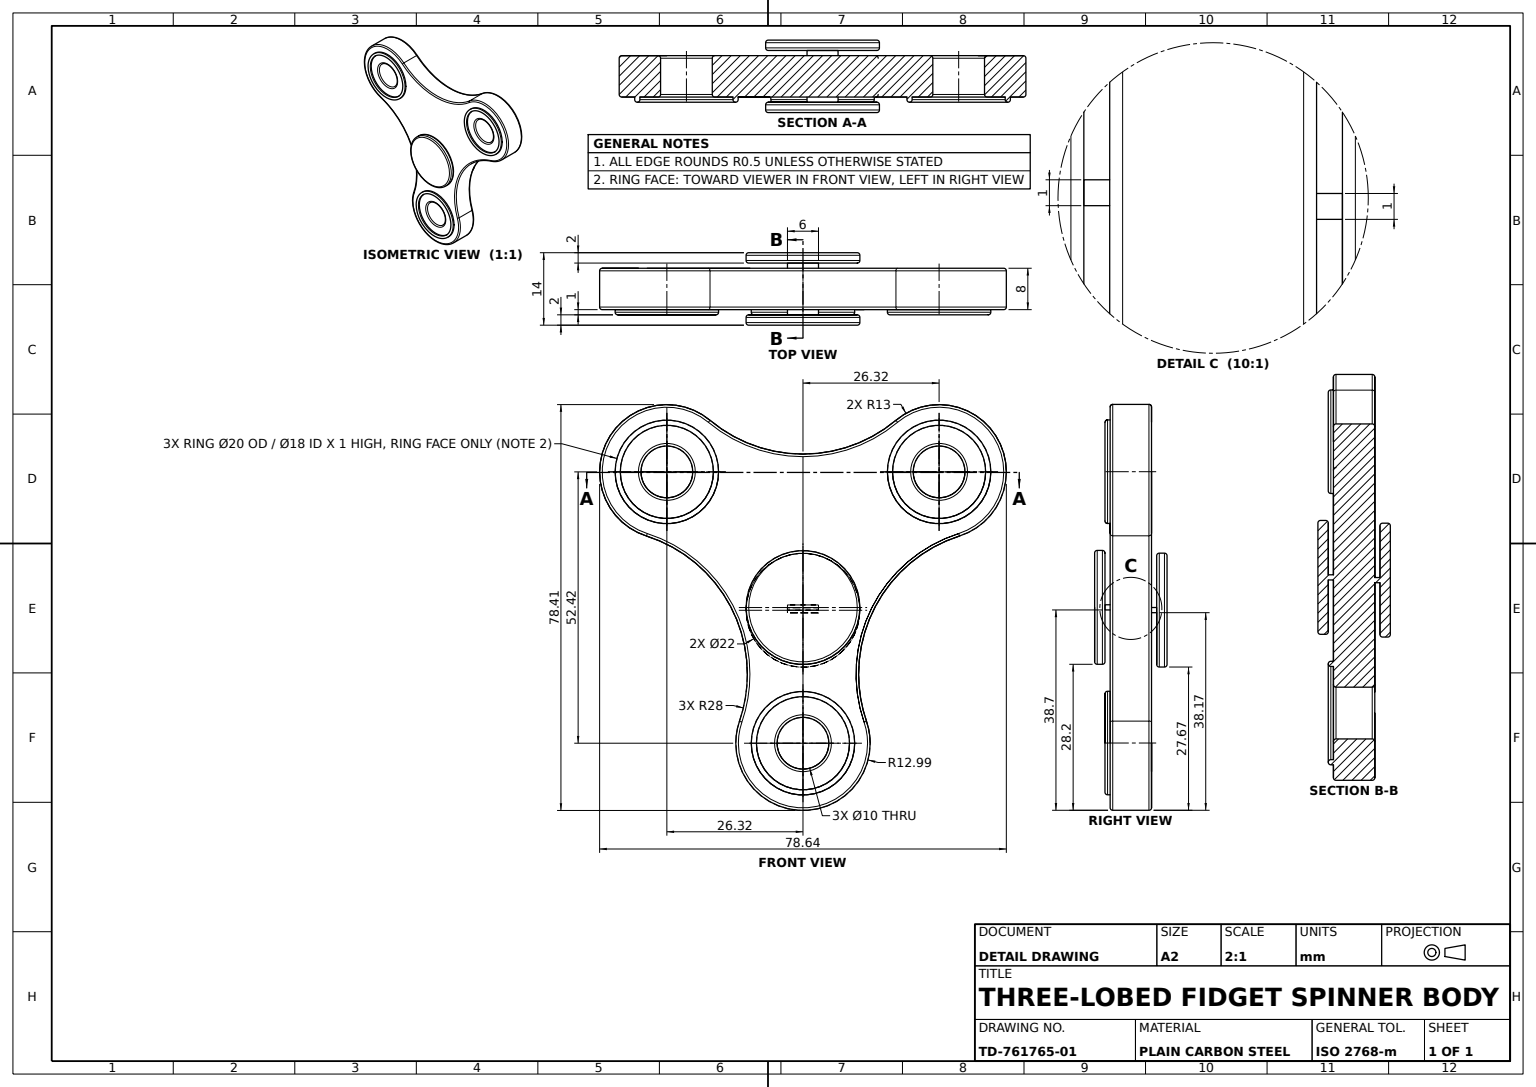
solid
v1 (-3,1.181214,0)
v2 (3,1.181214,0)
e1 v1 v2 LINE
v3 (3,1.181214,-1)
e2 v3 v2 LINE
v4 (-3,1.181214,-1)
e3 v4 v3 LINE
e4 v4 v1 LINE
face PLANE(AX(P(3,1.181214,-1),D(0,-1,0),D(0,0,-1))) rev [e1 -e2 -e3 e4]
v5 (35.319974,27.417425,8)
v6 (17.319974,27.417425,8)
e5 v5 v6 CIRCLE(AX(P(26.319974,27.417425,8),D(0,0,-1),D(1,0,0)),9)
e6 v6 v5 CIRCLE(AX(P(26.319974,27.417425,8),D(0,0,-1),D(1,0,0)),9)
v7 (20.819974,27.417425,8)
v8 (31.819974,27.417425,8)
e7 v7 v8 CIRCLE(AX(P(26.319974,27.417425,8),D(0,0,-1),D(1,0,0)),5.5)
e8 v8 v7 CIRCLE(AX(P(26.319974,27.417425,8),D(0,0,-1),D(1,0,0)),5.5)
face PLANE(AX(P(-32.539106,7.883547,8),D(0,0,1),D(1,0,0))) [-e5 -e6] [e7 e8]
v9 (16.819974,27.417425,9)
v10 (35.819974,27.417425,9)
e9 v9 v10 CIRCLE(AX(P(26.319974,27.417425,9),D(0,0,1),D(1,0,0)),9.5)
v11 (16.319974,27.417425,8.5)
e10 v11 v9 CIRCLE(AX(P(16.819974,27.417425,8.5),D(0,1,0),D(-1,0,0)),0.5)
v12 (36.319974,27.417425,8.5)
e11 v12 v11 CIRCLE(AX(P(26.319974,27.417425,8.5),D(0,0,-1),D(1,0,0)),10)
e12 v12 v10 CIRCLE(AX(P(35.819974,27.417425,8.5),D(0,-1,0),D(0,0,-1)),0.5)
face TORUS(AX(P(26.319974,27.417425,8.5),D(0,0,1),D(1,0,0)),9.5,0.5) [-e9 -e10 -e11 e12]
v13 (21.319974,27.417425,7.5)
e13 v7 v13 CIRCLE(AX(P(20.819974,27.417425,7.5),D(0,1,0),D(-1,0,0)),0.5)
v14 (31.319974,27.417425,7.5)
e14 v14 v13 CIRCLE(AX(P(26.319974,27.417425,7.5),D(0,0,1),D(1,0,0)),5)
e15 v8 v14 CIRCLE(AX(P(31.819974,27.417425,7.5),D(0,-1,0),D(0,0,-1)),0.5)
face TORUS(AX(P(26.319974,27.417425,7.5),D(0,0,1),D(1,0,0)),5.5,0.5) [-e7 e13 -e14 -e15]
v15 (11,0.681214,-1.5)
v16 (-11,0.681214,-1.5)
e16 v15 v16 CIRCLE(AX(P(0,0.681214,-1.5),D(0,0,-1),D(-1,0,0)),11)
v17 (10.5,0.681214,-1)
e17 v17 v15 CIRCLE(AX(P(10.5,0.681214,-1.5),D(0,1,0),D(-1,0,0)),0.5)
v18 (-10.5,0.681214,-1)
e18 v18 v17 CIRCLE(AX(P(0,0.681214,-1),D(0,0,1),D(-1,0,0)),10.5)
e19 v18 v16 CIRCLE(AX(P(-10.5,0.681214,-1.5),D(0,-1,0),D(0,0,-1)),0.5)
face TORUS(AX(P(0,0.681214,-1.5),D(0,0,-1),D(-1,0,0)),10.5,0.5) [-e16 -e17 -e18 e19]
v19 (-11,1.21,10.5)
v20 (-11,1.21,9.5)
e20 v19 v20 LINE
v21 (11,1.21,9.5)
e21 v20 v21 CIRCLE(AX(P(0,1.21,9.5),D(0,0,1),D(1,0,0)),11)
v22 (11,1.21,10.5)
e22 v22 v21 LINE
e23 v22 v19 CIRCLE(AX(P(0,1.21,10.5),D(0,0,-1),D(1,0,0)),11)
face CYL(AX(P(0,1.21,11),D(0,0,-1),D(-1,0,0)),11) [e20 e21 -e22 e23]
v23 (-10.258238,-11.650331,0)
v24 (-30.112128,15.506524,0)
e24 v23 v24 CIRCLE(AX(P(-38.758238,-11.650331,0),D(0,0,1),D(1,0,0)),28.5)
v25 (-10.758238,-11.650331,0.5)
e25 v25 v23 CIRCLE(AX(P(-10.258238,-11.650331,0.5),D(0,-1,0),D(0,0,-1)),0.5)
v26 (-30.263814,15.030088,0.5)
e26 v26 v25 CIRCLE(AX(P(-38.758238,-11.650331,0.5),D(0,0,-1),D(1,0,0)),28)
e27 v24 v26 CIRCLE(AX(P(-30.112128,15.506524,0.5),D(-0.952872102,0.303372309,0),D(-0.303372309,-0.952872102,0)),0.5)
face TORUS(AX(P(-38.758238,-11.650331,0.5),D(0,0,1),D(1,0,0)),28.5,0.5) [-e24 -e25 -e26 -e27]
v27 (-11,0.681214,-2.5)
e28 v27 v16 LINE
e29 v16 v15 CIRCLE(AX(P(0,0.681214,-1.5),D(0,0,-1),D(-1,0,0)),11)
v28 (11,0.681214,-2.5)
e30 v28 v15 LINE
e31 v28 v27 CIRCLE(AX(P(0,0.681214,-2.5),D(0,0,1),D(-1,0,0)),11)
face CYL(AX(P(0,0.681214,-3),D(0,0,1),D(1,0,0)),11) [e28 e29 -e30 e31]
v29 (-16.819974,27.417425,9)
v30 (-35.819974,27.417425,9)
e32 v29 v30 CIRCLE(AX(P(-26.319974,27.417425,9),D(0,0,1),D(1,0,0)),9.5)
v31 (-16.319974,27.417425,8.5)
e33 v31 v29 CIRCLE(AX(P(-16.819974,27.417425,8.5),D(0,-1,0),D(0,0,-1)),0.5)
v32 (-36.319974,27.417425,8.5)
e34 v32 v31 CIRCLE(AX(P(-26.319974,27.417425,8.5),D(0,0,-1),D(1,0,0)),10)
e35 v32 v30 CIRCLE(AX(P(-35.819974,27.417425,8.5),D(0,1,0),D(-1,0,0)),0.5)
face TORUS(AX(P(-26.319974,27.417425,8.5),D(0,0,1),D(1,0,0)),9.5,0.5) [-e32 -e33 -e34 e35]
v33 (11.811845,-20.931595,8)
v34 (30.112128,15.506524,8)
e36 v33 v34 CIRCLE(AX(P(38.758238,-11.650331,8),D(0,0,-1),D(1,0,0)),28.5)
v35 (12.284588,-20.768766,7.5)
e37 v35 v33 CIRCLE(AX(P(11.811845,-20.931595,7.5),D(0.325658377,-0.945487505,0),D(0.945487505,0.325658377,0)),0.5)
v36 (10.758238,-11.650331,7.5)
e38 v36 v35 CIRCLE(AX(P(38.758238,-11.650331,7.5),D(0,0,1),D(1,0,0)),28)
v37 (30.263814,15.030088,7.5)
e39 v37 v36 CIRCLE(AX(P(38.758238,-11.650331,7.5),D(0,0,1),D(1,0,0)),28)
e40 v34 v37 CIRCLE(AX(P(30.112128,15.506524,7.5),D(0.952872102,0.303372309,0),D(-0.303372309,0.952872102,0)),0.5)
face TORUS(AX(P(38.758238,-11.650331,7.5),D(0,0,1),D(1,0,0)),28.5,0.5) [-e36 -e37 -e38 -e39 -e40]
v38 (10.5,1.21,11)
e41 v22 v38 CIRCLE(AX(P(10.5,1.21,10.5),D(0,-1,0),D(0,0,-1)),0.5)
v39 (-10.5,1.21,11)
e42 v39 v38 CIRCLE(AX(P(0,1.21,11),D(0,0,1),D(1,0,0)),10.5)
e43 v19 v39 CIRCLE(AX(P(-10.5,1.21,10.5),D(0,1,0),D(-1,0,0)),0.5)
face TORUS(AX(P(0,1.21,10.5),D(0,0,1),D(1,0,0)),10.5,0.5) [-e23 e41 -e42 -e43]
v40 (-31.319974,27.417425,0.5)
v41 (-21.319974,27.417425,0.5)
e44 v40 v41 CIRCLE(AX(P(-26.319974,27.417425,0.5),D(0,0,-1),D(1,0,0)),5)
v42 (-21.319974,27.417425,7.5)
e45 v41 v42 LINE
v43 (-31.319974,27.417425,7.5)
e46 v42 v43 CIRCLE(AX(P(-26.319974,27.417425,7.5),D(0,0,1),D(1,0,0)),5)
e47 v40 v43 LINE
face CYL(AX(P(-26.319974,27.417425,0),D(0,0,1),D(1,0,0)),5) rev [e44 e45 e46 -e47]
v44 (-17.974616,37.385123,0.5)
v45 (-18.295592,37.00175,0)
e48 v44 v45 CIRCLE(AX(P(-18.295592,37.00175,0.5),D(-0.766746016,0.64195058,0),D(-0.64195058,-0.766746016,0)),0.5)
v46 (17.974616,37.385123,0.5)
e49 v46 v44 CIRCLE(AX(P(0,58.854012,0.5),D(0,0,-1),D(1,0,0)),28)
v47 (18.295592,37.00175,0)
e50 v46 v47 CIRCLE(AX(P(18.295592,37.00175,0.5),D(-0.766746016,-0.64195058,0),D(0.64195058,-0.766746016,0)),0.5)
e51 v45 v47 CIRCLE(AX(P(0,58.854012,0),D(0,0,1),D(1,0,0)),28.5)
face TORUS(AX(P(0,58.854012,0.5),D(0,0,1),D(1,0,0)),28.5,0.5) [-e48 -e49 e50 -e51]
v48 (3,0.181214,-1)
e52 v3 v48 LINE
v49 (-3,0.181214,-1)
e53 v48 v49 LINE
e54 v49 v4 LINE
e55 v17 v18 CIRCLE(AX(P(0,0.681214,-1),D(0,0,1),D(-1,0,0)),10.5)
face PLANE(AX(P(0,0.681214,-1),D(0,0,-1),D(-1,0,0))) rev [e52 e53 e54 e3] [e18 e55]
v50 (-30.263814,15.030088,7.5)
v51 (-30.112128,15.506524,8)
e56 v50 v51 CIRCLE(AX(P(-30.112128,15.506524,7.5),D(-0.952872102,0.303372309,0),D(-0.303372309,-0.952872102,0)),0.5)
v52 (-18.295592,37.00175,8)
e57 v52 v51 CIRCLE(AX(P(-26.319974,27.417425,8),D(0,0,1),D(1,0,0)),12.5)
v53 (-17.974616,37.385123,7.5)
e58 v52 v53 CIRCLE(AX(P(-18.295592,37.00175,7.5),D(-0.766746016,0.64195058,0),D(-0.64195058,-0.766746016,0)),0.5)
v54 (-39.319974,27.417425,7.5)
e59 v54 v53 CIRCLE(AX(P(-26.319974,27.417425,7.5),D(0,0,-1),D(1,0,0)),13)
e60 v50 v54 CIRCLE(AX(P(-26.319974,27.417425,7.5),D(0,0,-1),D(1,0,0)),13)
face TORUS(AX(P(-26.319974,27.417425,7.5),D(0,0,1),D(1,0,0)),12.5,0.5) [e56 -e57 e58 -e59 -e60]
v55 (16.319974,27.417425,8)
e61 v11 v55 LINE
v56 (36.319974,27.417425,8)
e62 v55 v56 CIRCLE(AX(P(26.319974,27.417425,8),D(0,0,1),D(1,0,0)),10)
e63 v12 v56 LINE
face CYL(AX(P(26.319974,27.417425,9),D(0,0,-1),D(-1,0,0)),10) [e61 e62 -e63 e11]
v57 (10,-25,8.5)
v58 (10,-25,8)
e64 v57 v58 LINE
v59 (-10,-25,8.5)
e65 v57 v59 CIRCLE(AX(P(0,-25,8.5),D(0,0,-1),D(1,0,0)),10)
v60 (-10,-25,8)
e66 v59 v60 LINE
e67 v60 v58 CIRCLE(AX(P(0,-25,8),D(0,0,1),D(1,0,0)),10)
face CYL(AX(P(0,-25,9),D(0,0,-1),D(-1,0,0)),10) [-e64 e65 e66 e67]
e68 v38 v39 CIRCLE(AX(P(0,1.21,11),D(0,0,1),D(1,0,0)),10.5)
e69 v19 v22 CIRCLE(AX(P(0,1.21,10.5),D(0,0,-1),D(1,0,0)),11)
face TORUS(AX(P(0,1.21,10.5),D(0,0,1),D(1,0,0)),10.5,0.5) [e43 -e68 -e41 -e69]
v61 (-11.811845,-20.931595,0)
v62 (-12.284588,-20.768766,0.5)
e70 v61 v62 CIRCLE(AX(P(-11.811845,-20.931595,0.5),D(0.325658377,0.945487505,0),D(-0.945487505,0.325658377,0)),0.5)
e71 v25 v62 CIRCLE(AX(P(-38.758238,-11.650331,0.5),D(0,0,-1),D(1,0,0)),28)
e72 v61 v23 CIRCLE(AX(P(-38.758238,-11.650331,0),D(0,0,1),D(1,0,0)),28.5)
face TORUS(AX(P(-38.758238,-11.650331,0.5),D(0,0,1),D(1,0,0)),28.5,0.5) [e70 -e71 e25 -e72]
e73 v50 v26 LINE
v63 (-12.284588,-20.768766,7.5)
e74 v63 v62 LINE
v64 (-10.758238,-11.650331,7.5)
e75 v63 v64 CIRCLE(AX(P(-38.758238,-11.650331,7.5),D(0,0,1),D(1,0,0)),28)
e76 v64 v50 CIRCLE(AX(P(-38.758238,-11.650331,7.5),D(0,0,1),D(1,0,0)),28)
face CYL(AX(P(-38.758238,-11.650331,8),D(0,0,-1),D(-1,0,0)),28) rev [e73 e26 e71 -e74 e75 e76]
v65 (12.992862,-25,7.5)
v66 (12.492862,-25,8)
e77 v65 v66 CIRCLE(AX(P(12.492862,-25,7.5),D(0,-1,0),D(0,0,-1)),0.5)
e78 v35 v65 CIRCLE(AX(P(0,-25,7.5),D(0,0,-1),D(1,0,0)),12.992862)
e79 v66 v33 CIRCLE(AX(P(0,-25,8),D(0,0,1),D(1,0,0)),12.492862)
face TORUS(AX(P(0,-25,7.5),D(0,0,1),D(1,0,0)),12.492862,0.5) [-e77 -e78 e37 -e79]
v67 (17.319974,27.417425,8.5)
e80 v67 v6 LINE
v68 (35.319974,27.417425,8.5)
e81 v68 v5 LINE
e82 v68 v67 CIRCLE(AX(P(26.319974,27.417425,8.5),D(0,0,1),D(1,0,0)),9)
face CYL(AX(P(26.319974,27.417425,9),D(0,0,-1),D(-1,0,0)),9) rev [e80 e6 -e81 e82]
v69 (-17.319974,27.417425,8.5)
v70 (-35.319974,27.417425,8.5)
e83 v69 v70 CIRCLE(AX(P(-26.319974,27.417425,8.5),D(0,0,1),D(1,0,0)),9)
v71 (-35.319974,27.417425,8)
e84 v70 v71 LINE
v72 (-17.319974,27.417425,8)
e85 v72 v71 CIRCLE(AX(P(-26.319974,27.417425,8),D(0,0,1),D(1,0,0)),9)
e86 v69 v72 LINE
face CYL(AX(P(-26.319974,27.417425,9),D(0,0,-1),D(-1,0,0)),9) rev [e83 e84 -e85 -e86]
v73 (31.319974,27.417425,0.5)
v74 (21.319974,27.417425,0.5)
e87 v73 v74 CIRCLE(AX(P(26.319974,27.417425,0.5),D(0,0,-1),D(1,0,0)),5)
e88 v74 v13 LINE
e89 v13 v14 CIRCLE(AX(P(26.319974,27.417425,7.5),D(0,0,1),D(1,0,0)),5)
e90 v73 v14 LINE
face CYL(AX(P(26.319974,27.417425,0),D(0,0,1),D(1,0,0)),5) rev [e87 e88 e89 -e90]
v75 (17.974616,37.385123,7.5)
e91 v53 v75 CIRCLE(AX(P(0,58.854012,7.5),D(0,0,1),D(1,0,0)),28)
v76 (18.295592,37.00175,8)
e92 v76 v52 CIRCLE(AX(P(0,58.854012,8),D(0,0,-1),D(1,0,0)),28.5)
e93 v76 v75 CIRCLE(AX(P(18.295592,37.00175,7.5),D(-0.766746016,-0.64195058,0),D(0.64195058,-0.766746016,0)),0.5)
face TORUS(AX(P(0,58.854012,7.5),D(0,0,1),D(1,0,0)),28.5,0.5) [-e91 -e58 -e92 e93]
e94 v43 v42 CIRCLE(AX(P(-26.319974,27.417425,7.5),D(0,0,1),D(1,0,0)),5)
e95 v41 v40 CIRCLE(AX(P(-26.319974,27.417425,0.5),D(0,0,-1),D(1,0,0)),5)
face CYL(AX(P(-26.319974,27.417425,0),D(0,0,1),D(1,0,0)),5) rev [e94 -e45 e95 e47]
v77 (-20.819974,27.417425,8)
v78 (-31.819974,27.417425,8)
e96 v77 v78 CIRCLE(AX(P(-26.319974,27.417425,8),D(0,0,-1),D(1,0,0)),5.5)
e97 v77 v42 CIRCLE(AX(P(-20.819974,27.417425,7.5),D(0,-1,0),D(0,0,-1)),0.5)
e98 v78 v43 CIRCLE(AX(P(-31.819974,27.417425,7.5),D(0,1,0),D(-1,0,0)),0.5)
face TORUS(AX(P(-26.319974,27.417425,7.5),D(0,0,1),D(1,0,0)),5.5,0.5) [-e96 e97 -e94 -e98]
v79 (-5.5,-25,8)
v80 (-5,-25,7.5)
e99 v79 v80 CIRCLE(AX(P(-5.5,-25,7.5),D(0,1,0),D(-1,0,0)),0.5)
v81 (5,-25,7.5)
e100 v81 v80 CIRCLE(AX(P(0,-25,7.5),D(0,0,1),D(1,0,0)),5)
v82 (5.5,-25,8)
e101 v82 v81 CIRCLE(AX(P(5.5,-25,7.5),D(0,-1,0),D(0,0,-1)),0.5)
e102 v79 v82 CIRCLE(AX(P(0,-25,8),D(0,0,-1),D(1,0,0)),5.5)
face TORUS(AX(P(0,-25,7.5),D(0,0,1),D(1,0,0)),5.5,0.5) [e99 -e100 -e101 -e102]
e103 v29 v69 CIRCLE(AX(P(-16.819974,27.417425,8.5),D(0,-1,0),D(0,0,-1)),0.5)
e104 v30 v70 CIRCLE(AX(P(-35.819974,27.417425,8.5),D(0,1,0),D(-1,0,0)),0.5)
face TORUS(AX(P(-26.319974,27.417425,8.5),D(0,0,1),D(1,0,0)),9.5,0.5) [-e83 -e103 e32 e104]
v83 (39.319974,27.417425,7.5)
v84 (38.819974,27.417425,8)
e105 v83 v84 CIRCLE(AX(P(38.819974,27.417425,7.5),D(0,-1,0),D(0,0,-1)),0.5)
e106 v75 v83 CIRCLE(AX(P(26.319974,27.417425,7.5),D(0,0,-1),D(1,0,0)),13)
e107 v84 v76 CIRCLE(AX(P(26.319974,27.417425,8),D(0,0,1),D(1,0,0)),12.5)
face TORUS(AX(P(26.319974,27.417425,7.5),D(0,0,1),D(1,0,0)),12.5,0.5) [-e105 -e106 -e93 -e107]
v85 (-16.319974,27.417425,8)
v86 (-36.319974,27.417425,8)
e108 v85 v86 CIRCLE(AX(P(-26.319974,27.417425,8),D(0,0,1),D(1,0,0)),10)
e109 v32 v86 LINE
e110 v31 v85 LINE
face CYL(AX(P(-26.319974,27.417425,9),D(0,0,-1),D(-1,0,0)),10) [e108 -e109 e34 e110]
v87 (-12.992862,-25,7.5)
e111 v87 v63 CIRCLE(AX(P(0,-25,7.5),D(0,0,-1),D(1,0,0)),12.992862)
v88 (-12.992862,-25,0.5)
e112 v62 v88 CIRCLE(AX(P(0,-25,0.5),D(0,0,1),D(1,0,0)),12.992862)
e113 v87 v88 LINE
face CYL(AX(P(0,-25,8),D(0,0,-1),D(-1,0,0)),12.992862) [e111 e74 e112 -e113]
e114 v10 v9 CIRCLE(AX(P(26.319974,27.417425,9),D(0,0,1),D(1,0,0)),9.5)
e115 v11 v12 CIRCLE(AX(P(26.319974,27.417425,8.5),D(0,0,-1),D(1,0,0)),10)
face TORUS(AX(P(26.319974,27.417425,8.5),D(0,0,1),D(1,0,0)),9.5,0.5) [e10 -e114 -e12 -e115]
v89 (-20.819974,27.417425,0)
e116 v41 v89 CIRCLE(AX(P(-20.819974,27.417425,0.5),D(0,-1,0),D(0,0,-1)),0.5)
v90 (-31.819974,27.417425,0)
e117 v40 v90 CIRCLE(AX(P(-31.819974,27.417425,0.5),D(0,1,0),D(-1,0,0)),0.5)
e118 v89 v90 CIRCLE(AX(P(-26.319974,27.417425,0),D(0,0,1),D(1,0,0)),5.5)
face TORUS(AX(P(-26.319974,27.417425,0.5),D(0,0,1),D(1,0,0)),5.5,0.5) [-e116 -e44 e117 -e118]
v91 (-39.319974,27.417425,0.5)
e119 v91 v26 CIRCLE(AX(P(-26.319974,27.417425,0.5),D(0,0,1),D(1,0,0)),13)
e120 v44 v91 CIRCLE(AX(P(-26.319974,27.417425,0.5),D(0,0,1),D(1,0,0)),13)
e121 v24 v45 CIRCLE(AX(P(-26.319974,27.417425,0),D(0,0,-1),D(1,0,0)),12.5)
face TORUS(AX(P(-26.319974,27.417425,0.5),D(0,0,1),D(1,0,0)),12.5,0.5) [-e119 -e120 e48 -e121 e27]
v92 (9,-25,8)
v93 (-9,-25,8)
e122 v92 v93 CIRCLE(AX(P(0,-25,8),D(0,0,-1),D(1,0,0)),9)
v94 (-9,-25,8.5)
e123 v94 v93 LINE
v95 (9,-25,8.5)
e124 v94 v95 CIRCLE(AX(P(0,-25,8.5),D(0,0,1),D(1,0,0)),9)
e125 v95 v92 LINE
face CYL(AX(P(0,-25,9),D(0,0,-1),D(-1,0,0)),9) rev [e122 -e123 e124 e125]
v96 (12.992862,-25,0.5)
e126 v65 v96 LINE
v97 (12.284588,-20.768766,0.5)
e127 v96 v97 CIRCLE(AX(P(0,-25,0.5),D(0,0,1),D(1,0,0)),12.992862)
e128 v35 v97 LINE
face CYL(AX(P(0,-25,8),D(0,0,-1),D(-1,0,0)),12.992862) [e126 e127 -e128 e78]
e129 v82 v79 CIRCLE(AX(P(0,-25,8),D(0,0,-1),D(1,0,0)),5.5)
e130 v93 v92 CIRCLE(AX(P(0,-25,8),D(0,0,-1),D(1,0,0)),9)
face PLANE(AX(P(-32.539106,7.883547,8),D(0,0,1),D(1,0,0))) [e129 e102] [-e122 -e130]
e131 v31 v32 CIRCLE(AX(P(-26.319974,27.417425,8.5),D(0,0,-1),D(1,0,0)),10)
e132 v86 v85 CIRCLE(AX(P(-26.319974,27.417425,8),D(0,0,1),D(1,0,0)),10)
face CYL(AX(P(-26.319974,27.417425,9),D(0,0,-1),D(-1,0,0)),10) [e131 e109 e132 -e110]
v98 (-10.5,0.681214,-3)
v99 (10.5,0.681214,-3)
e133 v98 v99 CIRCLE(AX(P(0,0.681214,-3),D(0,0,-1),D(-1,0,0)),10.5)
e134 v99 v98 CIRCLE(AX(P(0,0.681214,-3),D(0,0,-1),D(-1,0,0)),10.5)
face PLANE(AX(P(0,0.681214,-3),D(0,0,-1),D(-1,0,0))) [e133 e134]
v100 (-9.5,-25,9)
v101 (9.5,-25,9)
e135 v100 v101 CIRCLE(AX(P(0,-25,9),D(0,0,1),D(1,0,0)),9.5)
e136 v101 v95 CIRCLE(AX(P(9.5,-25,8.5),D(0,-1,0),D(0,0,-1)),0.5)
e137 v100 v94 CIRCLE(AX(P(-9.5,-25,8.5),D(0,1,0),D(-1,0,0)),0.5)
face TORUS(AX(P(0,-25,8.5),D(0,0,1),D(1,0,0)),9.5,0.5) [e135 e136 -e124 -e137]
v102 (-5,-25,0.5)
e138 v102 v80 LINE
v103 (5,-25,0.5)
e139 v102 v103 CIRCLE(AX(P(0,-25,0.5),D(0,0,-1),D(1,0,0)),5)
e140 v103 v81 LINE
face CYL(AX(P(0,-25,0),D(0,0,1),D(1,0,0)),5) rev [e100 -e138 e139 e140]
v104 (3,1.71,9)
v105 (-3,1.71,9)
e141 v104 v105 LINE
v106 (3,1.71,8)
e142 v104 v106 LINE
v107 (-3,1.71,8)
e143 v106 v107 LINE
e144 v105 v107 LINE
face PLANE(AX(P(-3,1.71,9),D(0,-1,0),D(1,0,0))) rev [-e141 e142 e143 -e144]
v108 (30.263814,15.030088,0.5)
v109 (30.112128,15.506524,0)
e145 v108 v109 CIRCLE(AX(P(30.112128,15.506524,0.5),D(0.952872102,0.303372309,0),D(-0.303372309,0.952872102,0)),0.5)
v110 (38.819974,27.417425,0)
e146 v110 v109 CIRCLE(AX(P(26.319974,27.417425,0),D(0,0,-1),D(1,0,0)),12.5)
v111 (39.319974,27.417425,0.5)
e147 v110 v111 CIRCLE(AX(P(38.819974,27.417425,0.5),D(0,-1,0),D(0,0,-1)),0.5)
e148 v108 v111 CIRCLE(AX(P(26.319974,27.417425,0.5),D(0,0,1),D(1,0,0)),13)
face TORUS(AX(P(26.319974,27.417425,0.5),D(0,0,1),D(1,0,0)),12.5,0.5) [e145 -e146 e147 -e148]
e149 v56 v55 CIRCLE(AX(P(26.319974,27.417425,8),D(0,0,1),D(1,0,0)),10)
face CYL(AX(P(26.319974,27.417425,9),D(0,0,-1),D(-1,0,0)),10) [e115 e63 e149 -e61]
e150 v59 v100 CIRCLE(AX(P(-9.5,-25,8.5),D(0,1,0),D(-1,0,0)),0.5)
e151 v57 v101 CIRCLE(AX(P(9.5,-25,8.5),D(0,-1,0),D(0,0,-1)),0.5)
face TORUS(AX(P(0,-25,8.5),D(0,0,1),D(1,0,0)),9.5,0.5) [-e150 -e65 e151 -e135]
v112 (-3,0.181214,0)
e152 v49 v112 LINE
e153 v112 v1 LINE
face PLANE(AX(P(-3,1.181214,-1),D(1,0,0),D(0,1,0))) rev [-e54 e152 e153 -e4]
e154 v27 v98 CIRCLE(AX(P(-10.5,0.681214,-2.5),D(0,-1,0),D(0,0,-1)),0.5)
e155 v28 v99 CIRCLE(AX(P(10.5,0.681214,-2.5),D(0,1,0),D(-1,0,0)),0.5)
e156 v27 v28 CIRCLE(AX(P(0,0.681214,-2.5),D(0,0,1),D(-1,0,0)),11)
face TORUS(AX(P(0,0.681214,-2.5),D(0,0,-1),D(-1,0,0)),10.5,0.5) [e154 -e134 -e155 -e156]
e157 v54 v91 LINE
e158 v53 v44 LINE
face CYL(AX(P(-26.319974,27.417425,8),D(0,0,-1),D(-1,0,0)),13) [e120 -e157 e59 e158]
e159 v101 v100 CIRCLE(AX(P(0,-25,9),D(0,0,1),D(1,0,0)),9.5)
e160 v95 v94 CIRCLE(AX(P(0,-25,8.5),D(0,0,1),D(1,0,0)),9)
face TORUS(AX(P(0,-25,8.5),D(0,0,1),D(1,0,0)),9.5,0.5) [e159 e137 -e160 -e136]
e161 v65 v87 CIRCLE(AX(P(0,-25,7.5),D(0,0,-1),D(1,0,0)),12.992862)
v113 (-12.492862,-25,8)
e162 v113 v66 CIRCLE(AX(P(0,-25,8),D(0,0,1),D(1,0,0)),12.492862)
e163 v87 v113 CIRCLE(AX(P(-12.492862,-25,7.5),D(0,1,0),D(-1,0,0)),0.5)
face TORUS(AX(P(0,-25,7.5),D(0,0,1),D(1,0,0)),12.492862,0.5) [-e161 e77 -e162 -e163]
face CYL(AX(P(-26.319974,27.417425,8),D(0,0,-1),D(-1,0,0)),13) [e60 e157 e119 -e73]
v114 (-10.258238,-11.650331,8)
e164 v51 v114 CIRCLE(AX(P(-38.758238,-11.650331,8),D(0,0,-1),D(1,0,0)),28.5)
e165 v114 v64 CIRCLE(AX(P(-10.258238,-11.650331,7.5),D(0,-1,0),D(0,0,-1)),0.5)
face TORUS(AX(P(-38.758238,-11.650331,7.5),D(0,0,1),D(1,0,0)),28.5,0.5) [-e164 -e56 -e76 -e165]
e166 v59 v57 CIRCLE(AX(P(0,-25,8.5),D(0,0,-1),D(1,0,0)),10)
face TORUS(AX(P(0,-25,8.5),D(0,0,1),D(1,0,0)),9.5,0.5) [-e166 e150 -e159 -e151]
v115 (10.758238,-11.650331,0.5)
e167 v97 v115 CIRCLE(AX(P(38.758238,-11.650331,0.5),D(0,0,-1),D(1,0,0)),28)
e168 v36 v115 LINE
face CYL(AX(P(38.758238,-11.650331,8),D(0,0,-1),D(-1,0,0)),28) rev [e167 -e168 e38 e128]
face CYL(AX(P(0,-25,9),D(0,0,-1),D(-1,0,0)),9) rev [e130 -e125 e160 e123]
e169 v103 v102 CIRCLE(AX(P(0,-25,0.5),D(0,0,-1),D(1,0,0)),5)
v116 (5.5,-25,0)
e170 v103 v116 CIRCLE(AX(P(5.5,-25,0.5),D(0,-1,0),D(0,0,-1)),0.5)
v117 (-5.5,-25,0)
e171 v117 v116 CIRCLE(AX(P(0,-25,0),D(0,0,1),D(1,0,0)),5.5)
e172 v102 v117 CIRCLE(AX(P(-5.5,-25,0.5),D(0,1,0),D(-1,0,0)),0.5)
face TORUS(AX(P(0,-25,0.5),D(0,0,1),D(1,0,0)),5.5,0.5) [-e169 e170 -e171 -e172]
v118 (3,0.71,8)
e173 v118 v106 LINE
v119 (3,0.71,9)
e174 v119 v104 LINE
e175 v119 v118 LINE
face PLANE(AX(P(3,1.71,9),D(-1,0,0),D(0,-1,0))) rev [e173 -e142 -e174 e175]
v120 (12.492862,-25,0)
e176 v120 v96 CIRCLE(AX(P(12.492862,-25,0.5),D(0,-1,0),D(0,0,-1)),0.5)
e177 v88 v96 CIRCLE(AX(P(0,-25,0.5),D(0,0,1),D(1,0,0)),12.992862)
v121 (-12.492862,-25,0)
e178 v121 v88 CIRCLE(AX(P(-12.492862,-25,0.5),D(0,1,0),D(-1,0,0)),0.5)
e179 v120 v121 CIRCLE(AX(P(0,-25,0),D(0,0,-1),D(1,0,0)),12.492862)
face TORUS(AX(P(0,-25,0.5),D(0,0,1),D(1,0,0)),12.492862,0.5) [e176 -e177 -e178 -e179]
e180 v78 v77 CIRCLE(AX(P(-26.319974,27.417425,8),D(0,0,-1),D(1,0,0)),5.5)
e181 v71 v72 CIRCLE(AX(P(-26.319974,27.417425,8),D(0,0,1),D(1,0,0)),9)
face PLANE(AX(P(-32.539106,7.883547,8),D(0,0,1),D(1,0,0))) [e180 e96] [e181 e85]
face TORUS(AX(P(0,0.681214,-1.5),D(0,0,-1),D(-1,0,0)),10.5,0.5) [e17 -e29 -e19 -e55]
e182 v70 v69 CIRCLE(AX(P(-26.319974,27.417425,8.5),D(0,0,1),D(1,0,0)),9)
face CYL(AX(P(-26.319974,27.417425,9),D(0,0,-1),D(-1,0,0)),9) rev [-e181 -e84 e182 e86]
e183 v9 v67 CIRCLE(AX(P(16.819974,27.417425,8.5),D(0,1,0),D(-1,0,0)),0.5)
e184 v10 v68 CIRCLE(AX(P(35.819974,27.417425,8.5),D(0,-1,0),D(0,0,-1)),0.5)
face TORUS(AX(P(26.319974,27.417425,8.5),D(0,0,1),D(1,0,0)),9.5,0.5) [e114 e183 -e82 -e184]
v122 (-3,0.71,8)
e185 v107 v122 LINE
v123 (-3,0.71,9)
e186 v123 v122 LINE
e187 v105 v123 LINE
face PLANE(AX(P(-3,1.71,9),D(1,0,0),D(0,1,0))) rev [e185 -e186 -e187 e144]
e188 v21 v20 CIRCLE(AX(P(0,1.21,9.5),D(0,0,1),D(1,0,0)),11)
face CYL(AX(P(0,1.21,11),D(0,0,-1),D(-1,0,0)),11) [e188 -e20 e69 e22]
e189 v80 v81 CIRCLE(AX(P(0,-25,7.5),D(0,0,1),D(1,0,0)),5)
face CYL(AX(P(0,-25,0),D(0,0,1),D(1,0,0)),5) rev [-e140 e169 e138 e189]
face TORUS(AX(P(26.319974,27.417425,7.5),D(0,0,1),D(1,0,0)),5.5,0.5) [-e89 -e13 -e8 e15]
v124 (-11.811845,-20.931595,8)
e190 v63 v124 CIRCLE(AX(P(-11.811845,-20.931595,7.5),D(0.325658377,0.945487505,0),D(-0.945487505,0.325658377,0)),0.5)
e191 v114 v124 CIRCLE(AX(P(-38.758238,-11.650331,8),D(0,0,-1),D(1,0,0)),28.5)
face TORUS(AX(P(-38.758238,-11.650331,7.5),D(0,0,1),D(1,0,0)),28.5,0.5) [-e75 e190 -e191 e165]
e192 v67 v68 CIRCLE(AX(P(26.319974,27.417425,8.5),D(0,0,1),D(1,0,0)),9)
face TORUS(AX(P(26.319974,27.417425,8.5),D(0,0,1),D(1,0,0)),9.5,0.5) [-e192 -e183 e9 e184]
face PLANE(AX(P(0,1.21,11),D(0,0,1),D(1,0,0))) [e42 e68]
e193 v90 v89 CIRCLE(AX(P(-26.319974,27.417425,0),D(0,0,1),D(1,0,0)),5.5)
face TORUS(AX(P(-26.319974,27.417425,0.5),D(0,0,1),D(1,0,0)),5.5,0.5) [-e117 -e95 e116 -e193]
v125 (3,0.181214,0)
e194 v125 v112 LINE
e195 v2 v125 LINE
e196 v116 v117 CIRCLE(AX(P(0,-25,0),D(0,0,1),D(1,0,0)),5.5)
v126 (11.811845,-20.931595,0)
e197 v126 v120 CIRCLE(AX(P(0,-25,0),D(0,0,-1),D(1,0,0)),12.492862)
e198 v121 v61 CIRCLE(AX(P(0,-25,0),D(0,0,-1),D(1,0,0)),12.492862)
e199 v47 v110 CIRCLE(AX(P(26.319974,27.417425,0),D(0,0,-1),D(1,0,0)),12.5)
e200 v109 v126 CIRCLE(AX(P(38.758238,-11.650331,0),D(0,0,1),D(1,0,0)),28.5)
v127 (31.819974,27.417425,0)
v128 (20.819974,27.417425,0)
e201 v127 v128 CIRCLE(AX(P(26.319974,27.417425,0),D(0,0,1),D(1,0,0)),5.5)
e202 v128 v127 CIRCLE(AX(P(26.319974,27.417425,0),D(0,0,1),D(1,0,0)),5.5)
face PLANE(AX(P(-32.539106,7.883547,0),D(0,0,1),D(1,0,0))) rev [-e153 -e194 -e195 -e1] [e196 e171] [e197 e179 e198 e72 e24 e121 e51 e199 e146 e200] [e193 e118] [e201 e202]
v129 (-10.5,1.21,9)
e203 v129 v20 CIRCLE(AX(P(-10.5,1.21,9.5),D(0,1,0),D(-1,0,0)),0.5)
v130 (10.5,1.21,9)
e204 v130 v129 CIRCLE(AX(P(0,1.21,9),D(0,0,-1),D(1,0,0)),10.5)
e205 v130 v21 CIRCLE(AX(P(10.5,1.21,9.5),D(0,-1,0),D(0,0,-1)),0.5)
face TORUS(AX(P(0,1.21,9.5),D(0,0,1),D(1,0,0)),10.5,0.5) [-e203 -e204 e205 -e21]
e206 v74 v73 CIRCLE(AX(P(26.319974,27.417425,0.5),D(0,0,-1),D(1,0,0)),5)
face CYL(AX(P(26.319974,27.417425,0),D(0,0,1),D(1,0,0)),5) rev [e14 -e88 e206 e90]
e207 v73 v127 CIRCLE(AX(P(31.819974,27.417425,0.5),D(0,-1,0),D(0,0,-1)),0.5)
e208 v74 v128 CIRCLE(AX(P(20.819974,27.417425,0.5),D(0,1,0),D(-1,0,0)),0.5)
face TORUS(AX(P(26.319974,27.417425,0.5),D(0,0,1),D(1,0,0)),5.5,0.5) [-e201 -e207 -e206 e208]
face CYL(AX(P(26.319974,27.417425,9),D(0,0,-1),D(-1,0,0)),9) rev [e192 e81 e5 -e80]
e209 v123 v119 LINE
e210 v122 v118 LINE
face PLANE(AX(P(-3,0.71,9),D(0,1,0),D(-1,0,0))) rev [-e209 e186 e210 -e175]
e211 v30 v29 CIRCLE(AX(P(-26.319974,27.417425,9),D(0,0,1),D(1,0,0)),9.5)
face TORUS(AX(P(-26.319974,27.417425,8.5),D(0,0,1),D(1,0,0)),9.5,0.5) [e33 -e211 -e35 -e131]
face TORUS(AX(P(0,-25,0.5),D(0,0,1),D(1,0,0)),5.5,0.5) [-e196 -e170 -e139 e172]
e212 v126 v97 CIRCLE(AX(P(11.811845,-20.931595,0.5),D(0.325658377,-0.945487505,0),D(0.945487505,0.325658377,0)),0.5)
face TORUS(AX(P(0,-25,0.5),D(0,0,1),D(1,0,0)),12.492862,0.5) [e212 -e127 -e176 -e197]
e213 v34 v84 CIRCLE(AX(P(26.319974,27.417425,8),D(0,0,1),D(1,0,0)),12.5)
e214 v83 v37 CIRCLE(AX(P(26.319974,27.417425,7.5),D(0,0,-1),D(1,0,0)),13)
face TORUS(AX(P(26.319974,27.417425,7.5),D(0,0,1),D(1,0,0)),12.5,0.5) [-e213 e40 -e214 e105]
e215 v37 v108 LINE
e216 v111 v46 CIRCLE(AX(P(26.319974,27.417425,0.5),D(0,0,1),D(1,0,0)),13)
e217 v75 v46 LINE
face CYL(AX(P(26.319974,27.417425,8),D(0,0,-1),D(-1,0,0)),13) [e106 e214 e215 e148 e216 -e217]
face CYL(AX(P(0,58.854012,8),D(0,0,-1),D(-1,0,0)),28) rev [e49 -e158 e91 e217]
face TORUS(AX(P(26.319974,27.417425,0.5),D(0,0,1),D(1,0,0)),12.5,0.5) [-e216 -e147 -e199 -e50]
e218 v115 v108 CIRCLE(AX(P(38.758238,-11.650331,0.5),D(0,0,-1),D(1,0,0)),28)
face TORUS(AX(P(38.758238,-11.650331,0.5),D(0,0,1),D(1,0,0)),28.5,0.5) [-e218 -e167 -e212 -e200 -e145]
face TORUS(AX(P(0,-25,7.5),D(0,0,1),D(1,0,0)),5.5,0.5) [-e129 e101 -e189 -e99]
face CYL(AX(P(38.758238,-11.650331,8),D(0,0,-1),D(-1,0,0)),28) rev [-e215 e39 e168 e218]
e219 v129 v130 CIRCLE(AX(P(0,1.21,9),D(0,0,-1),D(1,0,0)),10.5)
face PLANE(AX(P(0,1.21,9),D(0,0,1),D(1,0,0))) rev [e141 e187 e209 e174] [e204 e219]
face CYL(AX(P(0,0.681214,-3),D(0,0,1),D(1,0,0)),11) [e16 -e28 e156 e30]
e220 v124 v113 CIRCLE(AX(P(0,-25,8),D(0,0,1),D(1,0,0)),12.492862)
e221 v58 v60 CIRCLE(AX(P(0,-25,8),D(0,0,1),D(1,0,0)),10)
face PLANE(AX(P(-32.539106,7.883547,8),D(0,0,1),D(1,0,0))) [e213 e107 e92 e57 e164 e191 e220 e162 e79 e36] [-e149 -e62] [-e173 -e210 -e185 -e143] [-e221 -e67] [-e108 -e132]
face TORUS(AX(P(0,0.681214,-2.5),D(0,0,-1),D(-1,0,0)),10.5,0.5) [-e31 e155 -e133 -e154]
face TORUS(AX(P(0,-25,0.5),D(0,0,1),D(1,0,0)),12.492862,0.5) [-e198 e178 -e112 -e70]
face TORUS(AX(P(-26.319974,27.417425,7.5),D(0,0,1),D(1,0,0)),5.5,0.5) [-e46 -e97 -e180 e98]
face TORUS(AX(P(-26.319974,27.417425,8.5),D(0,0,1),D(1,0,0)),9.5,0.5) [e211 e103 -e182 -e104]
e222 v48 v125 LINE
face PLANE(AX(P(3,0.181214,-1),D(0,1,0),D(0,0,1))) rev [e222 e194 -e152 -e53]
face PLANE(AX(P(3,1.181214,-1),D(-1,0,0),D(0,-1,0))) rev [e2 e195 -e222 -e52]
face CYL(AX(P(0,-25,8),D(0,0,-1),D(-1,0,0)),12.992862) [e161 e113 e177 -e126]
face TORUS(AX(P(26.319974,27.417425,0.5),D(0,0,1),D(1,0,0)),5.5,0.5) [e207 -e202 -e208 -e87]
face TORUS(AX(P(0,-25,7.5),D(0,0,1),D(1,0,0)),12.492862,0.5) [-e111 e163 -e220 -e190]
face TORUS(AX(P(0,1.21,9.5),D(0,0,1),D(1,0,0)),10.5,0.5) [e203 -e188 -e205 -e219]
face CYL(AX(P(0,-25,9),D(0,0,-1),D(-1,0,0)),10) [-e66 e166 e64 e221]
